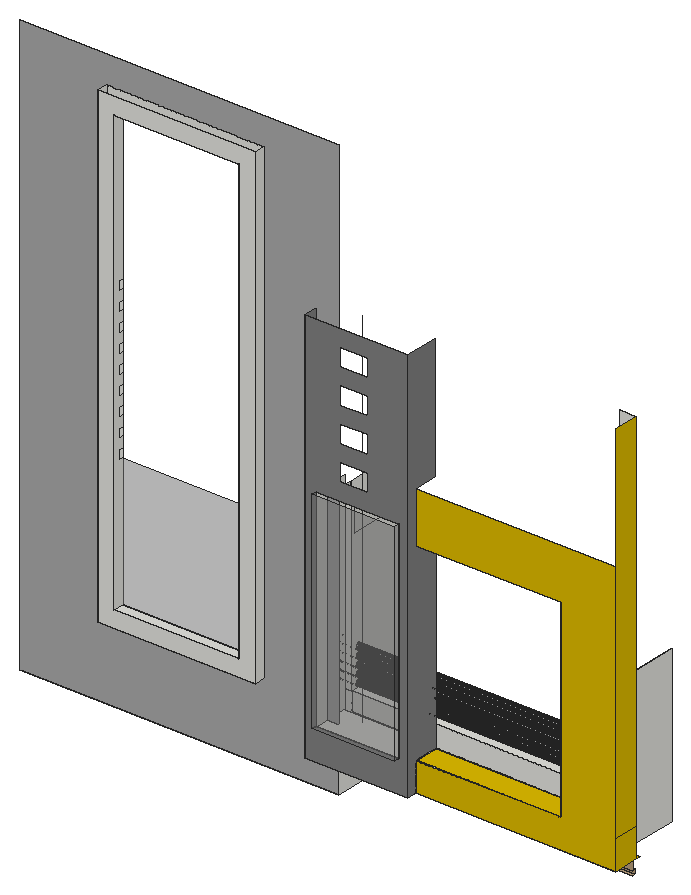
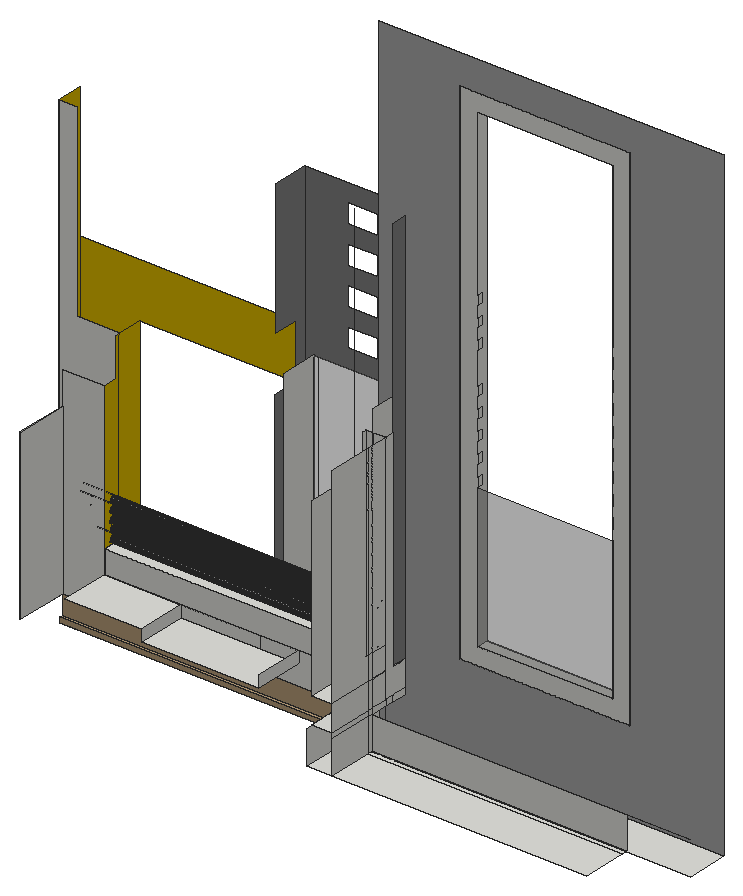
# SketchUp Ruby script. Lengths in inches.
U = 1.inch
M = Sketchup.active_model
def pt(a) = Geom::Point3d.new(a.map { |v| v * U })
def face(e, loops, mat)
  f = e.add_face(loops[0].map { |a| pt(a) })
  loops[1..].each { |l| e.add_face(l.map { |a| pt(a) }).erase! }
  f.material = f.back_material = mat if mat
  f
end
# faces: each face lists its corners as indices into pts; further lists are holes
def faces(e, pts, list, mat = nil) = list.each { |f| face(e, (f[0].is_a?(Array) ? f : [f]).map { |l| l.map { |i| pts[i] } }, mat) }
# xy, xz, yz: faces in a plane at the given z, y or x. An outline is a flat list of corners, or four numbers for a rectangle; further outlines are holes
def ring(l) = l.size == 4 ? [[l[0], l[1]], [l[2], l[1]], [l[2], l[3]], [l[0], l[3]]] : l.each_slice(2).to_a
def flat(e, list, mat, &to3) = list.each { |f| face(e, (f[0].is_a?(Array) ? f : [f]).map { |l| ring(l).map { |u, v| to3.(u, v) } }, mat) }
def xy(e, z, list, mat = nil) = flat(e, list, mat) { |x, y| [x, y, z] }
def xz(e, y, list, mat = nil) = flat(e, list, mat) { |x, z| [x, y, z] }
def yz(e, x, list, mat = nil) = flat(e, list, mat) { |y, z| [x, y, z] }
def lines(e, pts, list) = list.each { |a, b| e.add_line(pt(pts[a]), pt(pts[b])) }
# prism: a flat outline (further loops are holes) pulled along v
def prism(e, loops, v, mat = nil)
  f = face(e, loops, mat); d = Geom::Vector3d.new(v.map { |x| x * U })
  f.pushpull(f.normal.samedirection?(d) ? d.length : -d.length)
end
def box(e, o, s, mat = nil) = prism(e, [[o, [o[0] + s[0], o[1], o[2]], [o[0] + s[0], o[1] + s[1], o[2]], [o[0], o[1] + s[1], o[2]]]], [0, 0, s[2]], mat)
def at(x, y, z, deg = 0) = Geom::Transformation.translation(pt([x, y, z])) * Geom::Transformation.rotation(ORIGIN, Z_AXIS, deg.degrees)
def axes(o, x, y, z) = Geom::Transformation.new([*x, 0, *y, 0, *z, 0, *pt(o).to_a, 1])
def part(name) = M.definitions.add(name)
# library, detail: a bought-in or finely detailed component or shape, given as its bounding box
def library(name, o, s) = part(name).tap { |d| box(d.entities, o, s) }
def detail(e, o, s) = box(e.add_group.entities, o, s)
def put(e, d, t, mat = nil) = e.add_instance(d, t).tap { |i| i.material = mat if mat }
def group(e, t, mat = nil) = e.add_group.tap { |g| g.transformation = t; g.material = mat if mat }.entities
root = M.entities
M.materials.add("[0035_Tan]").color = [183, 157, 122]
M.materials.add("[0046_Gold]").color = [221, 186, 0]
M.materials.add("[0132_LightGray]").color = [169, 169, 169]
M.materials.add("[0133_Gray]").color = [128, 128, 128]
M.materials.add("[Translucent Glass Gray]").color = [128, 128, 128]
M.materials["[Translucent Glass Gray]"].alpha = 0.5
xy(root,103.1875,[[106,49.06,282.09,70.06],[138.64,70.06,269.16,72.5],[138.64,70.06,269.16,95.5],[269.16,70.06,282.09,95.5]])
xy(root,106.125,[[282.09,68.06,428.8,70.06]],"[0035_Tan]")
xy(root,108.51,[[282.09,68.06,428.8,70.06]],"[0035_Tan]")
xy(root,120,[[269.16,41.62,269.16,49.06,282.09,49.06,282.09,61.06,326.02,61.06,326.02,41.62],[326.02,47.37,436.31,47.62],[269.16,49.06,279.43,56.62],[279.43,49.06,279.47,56.62],[279.43,49.06,279.47,56.62],
  [279.47,49.06,282.09,61.06],[269.16,56.62,279.43,61.06],[279.43,56.62,279.47,61.06],[269.16,61.06,279.43,70.06],[279.43,61.06,279.47,70.06],
  [279.47,61.06,282.09,70.06],[282.09,61.06,326.02,68.06],[282.09,68.06,288.87,70.06],[288.87,68.06,326.02,70.06],[326.02,68.06,405.67,70.06],
  [405.67,68.06,427.31,70.06],[427.31,68.06,427.68,70.06],[427.31,70.06,427.68,96.62]])
xy(root,120,[[326.02,47.62,436.31,61.06],[326.02,61.06,326.02,68.06,428.8,68.06,428.8,64.12,436.31,64.12,436.31,61.06]],"[0046_Gold]")
xy(root,123,[[269.16,49.06,279.43,61.06],[279.43,49.06,279.47,56.62],[279.43,56.62,279.47,61.06],[279.47,56.62,288.87,61.06],[288.87,56.62,326.02,61.06],
  [269.16,61.06,279.43,70.06],[279.43,61.06,279.47,70.06],[279.47,61.06,288.87,70.06],[269.16,70.06,279.43,95.5],[279.43,70.06,279.47,95.5]])
xy(root,130.21,[[306.51,61.06,366.51,95.5]])
xy(root,136,[[279.43,49.06,279.47,56.62],[279.43,56.62,279.47,61.06],[306.51,61.06,326.02,61.12],[326.02,61.06,366.51,61.12]])
xy(root,136.125,[[326.02,47.37,405.67,47.62],[405.67,47.62,436.31,48.18],[405.67,48.18,436.31,61.06]])
xy(root,136.125,[[326.02,47.62,405.67,61.06]],"[0046_Gold]")
xy(root,136.21,[[269.16,49.06,279.43,60.93],[279.43,49.06,279.47,60.93],[269.16,60.93,279.43,61.06],[279.43,60.93,279.47,61.06],[269.16,61.06,279.43,70.06],
  [279.43,61.06,279.47,70.06],[279.47,61.06,306.51,70.06],[306.51,61.06,326.02,61.12],[326.02,61.06,366.51,61.12],[366.51,61.06,405.67,70.06],
  [306.51,61.12,326.02,70.06],[326.02,61.12,366.51,70.06],[269.16,70.06,279.43,95.5],[279.43,70.06,279.47,95.5],[366.51,70.06,405.67,95.5]])
xy(root,137.77,[[275.6,41.62,321.29,61.06]])
xy(root,137.77,[[275.6,38.62,321.29,41.62]],"[Translucent Glass Gray]")
xy(root,146.15,[[153.79,43.06,240.72,49.06]])
xy(root,148.21,[[269.16,61.06,279.43,70.06],[279.43,61.06,405.67,70.06]])
xy(root,155.15,[[162.79,43.06,231.72,49.06]])
xz(root,38.62,[[275.6,137.77,321.29,253.9]],"[Translucent Glass Gray]")
xz(root,41.62,[[[269.16,120,326.02,339],[275.6,137.77,321.29,253.9],[288.75,320.14,303.875,330.2],[288.75,301.14,303.875,311.2],[288.75,282.14,303.875,292.2],[288.75,263.14,303.875,273.2]]],"[0133_Gray]")
xz(root,43.06,[[[153.79,146.15,240.72,408.9],[162.79,155.15,231.72,399.9]]])
xz(root,47.37,[[326.02,120,436.31,120,436.31,270.5625,326.02,270.5625,326.02,242.5,405.67,242.5,405.67,136.125,326.02,136.125]],"[0046_Gold]")
xz(root,48.18,[[405.67,136.125,436.31,136.21]])
xz(root,49.06,[[269.16,120,279.43,123],[279.43,120,279.47,123],[269.16,123,279.43,136],[269.16,123,279.47,136.21],[279.43,123,279.47,136],
  [269.16,136,279.43,136.21],[279.43,136,279.47,136.21],[[153.79,146.15,240.72,408.9],[162.79,155.15,231.72,399.9]]])
xz(root,49.06,[[[106,103.1875,282.09,424.32],[153.79,146.15,240.72,408.9],[269.16,120,279.47,123],[279.43,242.5,279.43,243,279.47,243,279.47,270.5625,279.43,270.5625,279.43,339,279.47,339,279.47,242.5],[269.16,136,279.47,136.21]]],"[0132_LightGray]")
xz(root,49.06,[[162.79,155.15,231.72,227.92]],"[Translucent Glass Gray]")
xz(root,60.93,[[269.16,136.21,279.43,148.21],[279.43,136.21,279.47,148.21],[269.16,148.21,279.43,243],[279.43,148.21,279.47,242.5]])
xz(root,61.06,[[269.16,120,269.5,123],[269.5,120,279.43,123],[279.43,120,279.47,123],[279.47,120,326.02,123],[269.16,123,269.5,136.21],
  [269.5,123,279.43,136.21],[279.43,123,279.47,136],[279.47,123,288.87,136],[288.87,123,288.87,136,306.51,136,306.51,130.21,326.02,130.21,326.02,123],[326.02,123,326.02,130.21,366.51,130.21,366.51,133.125,405.67,133.125,405.67,123],
  [306.51,130.21,326.02,136],[326.02,130.21,366.51,133.125],[326.02,133.125,366.51,136],[366.51,133.125,366.51,136,405.67,136,405.67,136.125,427.31,136.125,427.31,133.125],[366.51,133.125,405.67,136],
  [405.67,133.125,427.31,136],[279.43,136,288.87,136.21],[288.87,136,306.51,136.21],[306.51,136,326.02,136.21],[326.02,136,366.51,136.125],
  [366.51,136,405.67,136.125],[405.67,136,427.31,136.125],[427.31,136,436.31,136.125],[326.02,136.125,366.51,136.21],[366.51,136.125,405.67,136.21],
  [405.67,136.125,427.31,136.21],[427.31,136.125,436.31,136.21],[269.16,136.21,269.5,148.21],[269.5,136.21,306.51,136.21,306.51,136.28,326.02,136.28,326.02,148.21,321.29,148.21,321.29,137.77,275.6,137.77,275.6,148.21,269.5,148.21],[306.51,136.21,326.02,136.28],
  [326.02,136.21,405.67,148.21],[405.67,136.21,405.67,243,427.31,243,427.31,339,436.31,339,436.31,136.21],[275.6,137.77,321.29,148.21],[269.16,148.21,269.5,243],[269.5,148.21,275.6,243],
  [275.6,148.21,279.43,243]])
xz(root,61.12,[[306.51,136,366.51,136.21]])
xz(root,68.06,[[282.09,108.51,428.8,120]],"[0035_Tan]")
xz(root,70.06,[[138.64,103.1875,269.16,120],[269.16,103.1875,279.43,120],[269.16,120,279.43,123],[279.43,120,288.87,123],[288.87,120,326.02,120,326.02,136.21,279.43,136.21,279.43,123,288.87,123],
  [326.02,120,405.67,136.21],[405.67,120,427.31,222.49],[427.31,120,427.68,205.375],[269.16,123,279.43,136.21],[269.16,136.21,279.43,148.21],
  [279.43,136.21,405.67,148.21]])
xz(root,70.06,[[279.43,103.1875,282.09,103.1875,282.09,106.125,428.8,106.125,428.8,108.51,282.09,108.51,282.09,120,279.43,120]],"[0035_Tan]")
yz(root,153.79,[[43.06,146.15,49.06,408.9]])
yz(root,162.79,[[43.06,155.15,49.06,155.15,49.06,227.92,46.06,227.92,46.06,232.84,49.06,232.84,49.06,238.36,46.06,238.36,46.06,243.28,49.06,243.28,49.06,248.8,46.06,248.8,46.06,253.71,49.06,253.71,49.06,259.23,46.06,259.23,46.06,264.15,49.06,264.15,49.06,269.67,46.06,269.67,46.06,274.59,49.06,274.59,49.06,280.11,46.06,280.11,46.06,285.03,49.06,285.03,49.06,290.55,46.06,290.55,46.06,295.46,49.06,295.46,49.06,300.98,46.06,300.98,46.06,305.9,49.06,305.9,49.06,311.42,46.06,311.42,46.06,316.34,49.06,316.34,49.06,399.9,43.06,399.9]])
yz(root,231.72,[[43.06,155.15,43.06,399.9,49.06,399.9,49.06,316.34,46.06,316.34,46.06,311.42,49.06,311.42,49.06,305.9,46.06,305.9,46.06,300.98,49.06,300.98,49.06,295.46,46.06,295.46,46.06,290.55,49.06,290.55,49.06,274.59,46.06,274.59,46.06,269.67,49.06,269.67,49.06,264.15,46.06,264.15,46.06,259.23,49.06,259.23,49.06,253.71,46.06,253.71,46.06,248.8,49.06,248.8,49.06,243.28,46.06,243.28,46.06,238.36,49.06,238.36,49.06,232.84,46.06,232.84,46.06,227.92,49.06,227.92,49.06,155.15]])
yz(root,240.72,[[43.06,146.15,49.06,408.9]])
yz(root,269.16,[[70.06,103.1875,72.5,120],[72.5,103.1875,95.5,120],[49.06,120,56.62,123],[56.62,120,61.06,123],[61.06,120,70.06,123],
  [70.06,120,72.5,123],[72.5,120,95.5,123],[49.06,123,49.06,136.21,56.62,136.21,56.62,243,60.93,243,60.93,123],[49.06,123,56.62,136],[56.62,123,60.93,136],
  [60.93,123,61.06,136],[61.06,123,70.06,136],[70.06,123,72.5,136],[72.5,123,95.5,136],[49.06,136,56.62,136.21],
  [56.62,136,60.93,136.21],[60.93,136,61.06,136.21],[61.06,136,70.06,136.21],[70.06,136,72.5,136.21],[72.5,136,95.5,136.21],
  [56.62,136.21,60.93,243],[60.93,136.21,61.06,148.21],[61.06,136.21,70.06,148.21],[70.06,136.21,72.5,148.21],[72.5,136.21,95.5,136.21,95.5,243,73.87,243,73.87,148.21,72.5,148.21],
  [60.93,148.21,61.06,243],[61.06,148.21,70.06,243],[70.06,148.21,72.5,243],[72.5,148.21,73.87,243]])
yz(root,269.16,[[41.62,120,41.62,339,56.62,339,56.62,136.21,49.06,136.21,49.06,120]],"[0133_Gray]")
yz(root,275.6,[[41.62,137.77,61.06,253.9]])
yz(root,275.6,[[38.62,137.77,41.62,253.9]],"[Translucent Glass Gray]")
yz(root,279.43,[[49.06,120,61.06,123],[61.06,120,70.06,123],[49.06,123,56.62,136],[56.62,123,61.06,136],[61.06,123,70.06,136],
  [49.06,136,61.06,136.21],[61.06,136,70.06,136.21],[70.06,136.21,95.5,136.21,95.5,225.3125,62.68,225.3125,62.68,242.5,61.06,242.5,61.06,148.21,70.06,148.21]])
yz(root,279.47,[[49.06,120,56.62,123],[56.62,120,61.06,123],[49.06,123,56.62,136],[56.62,123,61.06,136]])
yz(root,282.09,[[49.06,103.1875,68.06,103.1875,68.06,106.125,70.06,106.125,70.06,103.1875,95.5,103.1875,95.5,120,70.06,120,70.06,108.51,68.06,108.51,68.06,120,49.06,120],[68.06,103.1875,70.06,106.125],[68.06,108.51,70.06,120]])
yz(root,306.51,[[61.06,130.21,95.5,130.21,95.5,136.21,61.12,136.21,61.12,136,61.06,136],[61.06,136,61.12,136.21]])
yz(root,321.29,[[41.62,137.77,61.06,253.9]])
yz(root,321.29,[[38.62,137.77,41.62,253.9]],"[Translucent Glass Gray]")
yz(root,326.02,[[47.37,120,47.62,123],[47.62,120,61.06,123],[47.37,123,47.62,130.21],[47.62,123,56.62,130.21],[56.62,123,61.06,130.21],
  [47.37,130.21,47.62,133.125],[47.62,130.21,56.62,133.125],[56.62,130.21,61.06,133.125],[47.37,133.125,47.62,136],[47.62,133.125,56.62,136],
  [56.62,133.125,61.06,136],[47.37,136,47.62,136.125],[47.62,136,56.62,136.125],[56.62,136,61.06,136.125]])
yz(root,326.02,[[41.62,120,47.37,120,47.37,136.125,61.06,136.125,61.06,242.5,47.37,242.5,47.37,270.5625,60.18,270.5625,60.18,339,41.62,339]],"[0133_Gray]")
yz(root,366.51,[[61.06,130.21,61.06,136,61.12,136,61.12,136.21,95.5,136.21,95.5,130.21],[61.06,136,61.12,136.21]])
yz(root,405.67,[[48.18,136.125,61.06,136.21],[61.06,136.21,70.06,148.21]])
yz(root,405.67,[[47.37,136.125,47.37,242.5,61.06,242.5,61.06,136.21,48.18,136.21,48.18,136.125],[61.06,148.21,61.06,242.5,62.68,242.5,62.68,222.49,70.06,222.49,70.06,148.21]],"[0046_Gold]")
yz(root,412.03,[[65.33,153.59,65.76,153.64,66.17,153.8125,66.52,154.08,66.79,154.43,66.96,154.84,67.01,155.27,66.96,155.71,66.79,156.12,66.52,156.47,66.17,156.74,65.76,156.9,65.33,156.96,64.89,156.9,64.48,156.74,64.13,156.47,63.87,156.12,63.7,155.71,63.64,155.27,63.7,154.84,63.87,154.43,64.13,154.08,64.48,153.8125,64.89,153.64]])
yz(root,417.47,[[65.33,162.59,65.76,162.64,66.17,162.8125,66.52,163.08,66.79,163.43,66.96,163.84,67.01,164.27,66.96,164.71,66.79,165.12,66.52,165.47,66.17,165.74,65.76,165.9,65.33,165.96,64.89,165.9,64.48,165.74,64.13,165.47,63.87,165.12,63.7,164.71,63.64,164.27,63.7,163.84,63.87,163.43,64.13,163.08,64.48,162.8125,64.89,162.64]])
yz(root,421.03,[[65.33,167.09,65.76,167.14,66.17,167.3125,66.52,167.58,66.79,167.93,66.96,168.34,67.01,168.77,66.96,169.21,66.79,169.62,66.52,169.97,66.17,170.24,65.76,170.4,65.33,170.46,64.89,170.4,64.48,170.24,64.13,169.97,63.87,169.62,63.7,169.21,63.64,168.77,63.7,168.34,63.87,167.93,64.13,167.58,64.48,167.3125,64.89,167.14]])
yz(root,427.31,[[70.06,120,96.62,205.375]])
yz(root,427.68,[[70.06,120,96.62,205.375]])
yz(root,436.31,[[47.37,120,61.06,136.125],[47.37,136.125,61.06,339]],"[0046_Gold]")
p = [[269.16,64.48,149.3125],[269.16,64.89,149.14],[405.67,64.89,149.14],[405.67,64.48,149.3125],[269.16,65.33,149.09],[405.67,65.33,149.09],
  [269.16,65.76,149.14],[405.67,65.76,149.14],[269.16,66.17,149.3125],[405.67,66.17,149.3125],[269.16,64.13,149.58],[405.67,64.13,149.58],
  [269.16,66.52,149.58],[405.67,66.52,149.58],[269.16,63.87,149.93],[405.67,63.87,149.93],[269.16,66.79,149.93],[405.67,66.79,149.93],
  [269.16,63.7,150.34],[405.67,63.7,150.34],[269.16,66.96,150.34],[405.67,66.96,150.34],[269.16,63.64,150.77],[405.67,63.64,150.77],
  [269.16,67.01,150.77],[405.67,67.01,150.77],[269.16,63.7,151.21],[405.67,63.7,151.21],[269.16,66.96,151.21],[405.67,66.96,151.21],
  [269.16,63.87,151.62],[405.67,63.87,151.62],[269.16,66.79,151.62],[405.67,66.79,151.62],[269.16,64.13,151.97],[405.67,64.13,151.97],
  [269.16,66.52,151.97],[405.67,66.52,151.97],[269.16,64.48,152.24],[405.67,64.48,152.24],[269.16,66.17,152.24],[405.67,66.17,152.24],
  [269.16,64.89,152.4],[405.67,64.89,152.4],[269.16,65.76,152.4],[405.67,65.76,152.4],[269.16,65.33,152.46],[405.67,65.33,152.46],
  [269.16,64.48,153.8125],[269.16,64.89,153.64],[412.03,64.89,153.64],[412.03,64.48,153.8125],[269.16,65.33,153.59],[412.03,65.33,153.59],
  [269.16,65.76,153.64],[412.03,65.76,153.64],[269.16,66.17,153.8125],[412.03,66.17,153.8125],[269.16,64.13,154.08],[412.03,64.13,154.08],
  [269.16,66.52,154.08],[412.03,66.52,154.08],[269.16,63.87,154.43],[412.03,63.87,154.43],[269.16,66.79,154.43],[412.03,66.79,154.43],
  [269.16,63.7,154.84],[412.03,63.7,154.84],[269.16,66.96,154.84],[412.03,66.96,154.84],[269.16,63.64,155.27],[412.03,63.64,155.27],
  [269.16,67.01,155.27],[412.03,67.01,155.27],[269.16,63.7,155.71],[412.03,63.7,155.71],[269.16,66.96,155.71],[412.03,66.96,155.71],
  [269.16,63.87,156.12],[412.03,63.87,156.12],[269.16,66.79,156.12],[412.03,66.79,156.12],[269.16,64.13,156.47],[412.03,64.13,156.47],
  [269.16,66.52,156.47],[412.03,66.52,156.47],[269.16,64.48,156.74],[412.03,64.48,156.74],[269.16,66.17,156.74],[412.03,66.17,156.74],
  [269.16,64.89,156.9],[412.03,64.89,156.9],[269.16,65.76,156.9],[412.03,65.76,156.9],[269.16,65.33,156.96],[412.03,65.33,156.96],
  [269.16,64.48,158.3125],[269.16,64.89,158.14],[405.67,64.89,158.14],[405.67,64.48,158.3125],[269.16,65.33,158.09],[405.67,65.33,158.09],
  [269.16,65.76,158.14],[405.67,65.76,158.14],[269.16,66.17,158.3125],[405.67,66.17,158.3125],[269.16,64.13,158.58],[405.67,64.13,158.58],
  [269.16,66.52,158.58],[405.67,66.52,158.58],[269.16,63.87,158.93],[405.67,63.87,158.93],[269.16,66.79,158.93],[405.67,66.79,158.93],
  [269.16,63.7,159.34],[405.67,63.7,159.34],[269.16,66.96,159.34],[405.67,66.96,159.34],[269.16,63.64,159.77],[405.67,63.64,159.77],
  [269.16,67.01,159.77],[405.67,67.01,159.77],[269.16,63.7,160.21],[405.67,63.7,160.21],[269.16,66.96,160.21],[405.67,66.96,160.21],
  [269.16,63.87,160.62],[405.67,63.87,160.62],[269.16,66.79,160.62],[405.67,66.79,160.62],[269.16,64.13,160.97],[405.67,64.13,160.97],
  [269.16,66.52,160.97],[405.67,66.52,160.97],[269.16,64.48,161.24],[405.67,64.48,161.24],[269.16,66.17,161.24],[405.67,66.17,161.24],
  [269.16,64.89,161.4],[405.67,64.89,161.4],[269.16,65.76,161.4],[405.67,65.76,161.4],[269.16,65.33,161.46],[405.67,65.33,161.46],
  [269.16,64.48,162.8125],[269.16,64.89,162.64],[417.47,64.89,162.64],[417.47,64.48,162.8125],[269.16,65.33,162.59],[417.47,65.33,162.59],
  [269.16,65.76,162.64],[417.47,65.76,162.64],[269.16,66.17,162.8125],[417.47,66.17,162.8125],[269.16,64.13,163.08],[417.47,64.13,163.08],
  [269.16,66.52,163.08],[417.47,66.52,163.08],[269.16,63.87,163.43],[417.47,63.87,163.43],[269.16,66.79,163.43],[417.47,66.79,163.43],
  [269.16,63.7,163.84],[417.47,63.7,163.84],[269.16,66.96,163.84],[417.47,66.96,163.84],[269.16,63.64,164.27],[417.47,63.64,164.27],
  [269.16,67.01,164.27],[417.47,67.01,164.27],[269.16,63.7,164.71],[417.47,63.7,164.71],[269.16,66.96,164.71],[417.47,66.96,164.71],
  [269.16,63.87,165.12],[417.47,63.87,165.12],[269.16,66.79,165.12],[417.47,66.79,165.12],[269.16,64.13,165.47],[417.47,64.13,165.47],
  [269.16,66.52,165.47],[417.47,66.52,165.47],[269.16,64.48,165.74],[417.47,64.48,165.74],[269.16,66.17,165.74],[417.47,66.17,165.74],
  [269.16,64.89,165.9],[417.47,64.89,165.9],[269.16,65.76,165.9],[417.47,65.76,165.9],[269.16,65.33,165.96],[417.47,65.33,165.96],
  [269.16,64.48,167.3125],[269.16,64.89,167.14],[421.03,64.89,167.14],[421.03,64.48,167.3125],[269.16,65.33,167.09],[421.03,65.33,167.09],
  [269.16,65.76,167.14],[421.03,65.76,167.14],[269.16,66.17,167.3125],[421.03,66.17,167.3125],[269.16,64.13,167.58],[421.03,64.13,167.58],
  [269.16,66.52,167.58],[421.03,66.52,167.58],[269.16,63.87,167.93],[421.03,63.87,167.93],[269.16,66.79,167.93],[421.03,66.79,167.93],
  [269.16,63.7,168.34],[421.03,63.7,168.34],[269.16,66.96,168.34],[421.03,66.96,168.34],[269.16,63.64,168.77],[421.03,63.64,168.77],
  [269.16,67.01,168.77],[421.03,67.01,168.77],[269.16,63.7,169.21],[421.03,63.7,169.21],[269.16,66.96,169.21],[421.03,66.96,169.21],
  [269.16,63.87,169.62],[421.03,63.87,169.62],[269.16,66.79,169.62],[421.03,66.79,169.62],[269.16,64.13,169.97],[421.03,64.13,169.97],
  [269.16,66.52,169.97],[421.03,66.52,169.97],[269.16,64.48,170.24],[421.03,64.48,170.24],[269.16,66.17,170.24],[421.03,66.17,170.24],
  [269.16,64.89,170.4],[421.03,64.89,170.4],[269.16,65.76,170.4],[421.03,65.76,170.4],[269.16,65.33,170.46],[421.03,65.33,170.46],
  [70.06,60.93,123],[70.06,61.06,123],[269.16,73.87,148.21],[279.43,73.87,148.21],[269.16,61.06,120],[269.16,61.06,103.1875],
  [288.87,61.06,136],[288.87,56.62,136],[288.87,56.62,123],[288.87,56.62,339],[106,70.06,120],[138.64,70.06,120],
  [326.02,47.62,136.125],[326.02,47.62,136.28]]
faces(root,p,[[0,1,2,3],[1,4,5,2],[4,6,7,5],[6,8,9,7],[10,0,3,11],[8,12,13,9],[14,10,11,15],[12,16,17,13],
  [18,14,15,19],[16,20,21,17],[22,18,19,23],[20,24,25,21],[26,22,23,27],[24,28,29,25],[30,26,27,31],[28,32,33,29],
  [34,30,31,35],[32,36,37,33],[38,34,35,39],[36,40,41,37],[42,38,39,43],[40,44,45,41],[46,42,43,47],[44,46,47,45],
  [48,49,50,51],[49,52,53,50],[52,54,55,53],[54,56,57,55],[58,48,51,59],[56,60,61,57],[62,58,59,63],[60,64,65,61],
  [66,62,63,67],[64,68,69,65],[70,66,67,71],[68,72,73,69],[74,70,71,75],[72,76,77,73],[78,74,75,79],[76,80,81,77],
  [82,78,79,83],[80,84,85,81],[86,82,83,87],[84,88,89,85],[90,86,87,91],[88,92,93,89],[94,90,91,95],[92,94,95,93],
  [96,97,98,99],[97,100,101,98],[100,102,103,101],[102,104,105,103],[106,96,99,107],[104,108,109,105],[110,106,107,111],[108,112,113,109],
  [114,110,111,115],[112,116,117,113],[118,114,115,119],[116,120,121,117],[122,118,119,123],[120,124,125,121],[126,122,123,127],[124,128,129,125],
  [130,126,127,131],[128,132,133,129],[134,130,131,135],[132,136,137,133],[138,134,135,139],[136,140,141,137],[142,138,139,143],[140,142,143,141],
  [144,145,146,147],[145,148,149,146],[148,150,151,149],[150,152,153,151],[154,144,147,155],[152,156,157,153],[158,154,155,159],[156,160,161,157],
  [162,158,159,163],[160,164,165,161],[166,162,163,167],[164,168,169,165],[170,166,167,171],[168,172,173,169],[174,170,171,175],[172,176,177,173],
  [178,174,175,179],[176,180,181,177],[182,178,179,183],[180,184,185,181],[186,182,183,187],[184,188,189,185],[190,186,187,191],[188,190,191,189],
  [192,193,194,195],[193,196,197,194],[196,198,199,197],[198,200,201,199],[202,192,195,203],[200,204,205,201],[206,202,203,207],[204,208,209,205],
  [210,206,207,211],[208,212,213,209],[214,210,211,215],[212,216,217,213],[218,214,215,219],[216,220,221,217],[222,218,219,223],[220,224,225,221],
  [226,222,223,227],[224,228,229,225],[230,226,227,231],[228,232,233,229],[234,230,231,235],[232,236,237,233],[238,234,235,239],[236,238,239,237]],"[0132_LightGray]")
lines(root,p,[[240,241],[242,243],[244,245],[246,247],[248,247],[247,249],[250,251],[252,253]])
